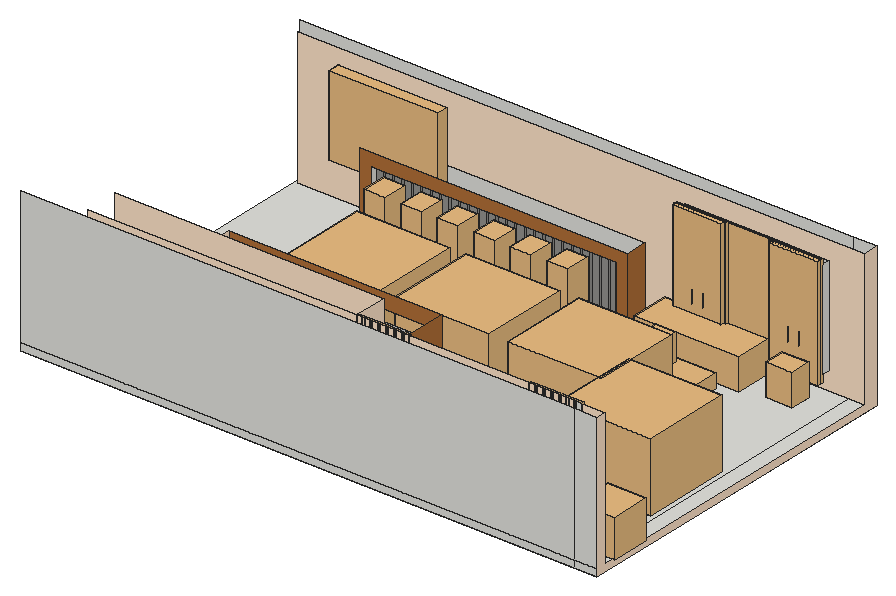
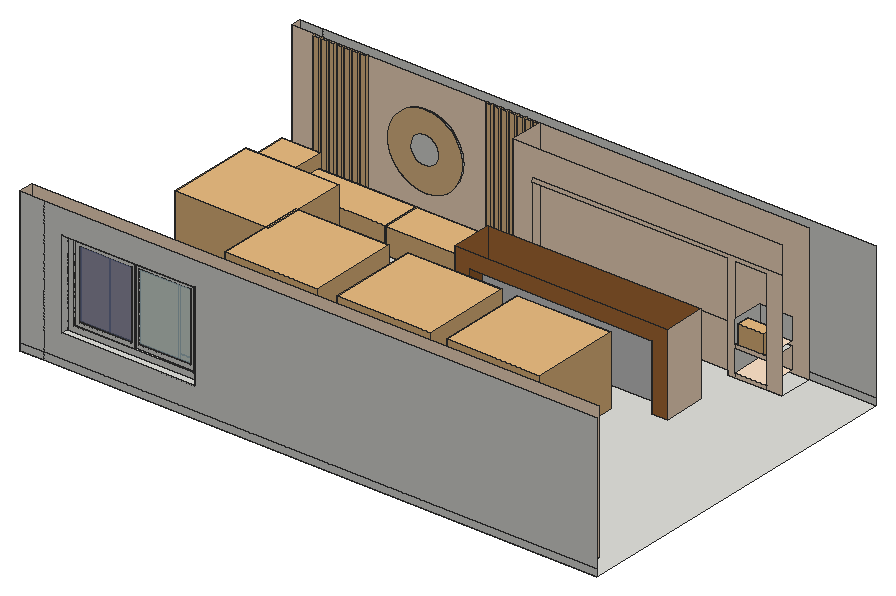
# SketchUp Ruby script. Lengths in inches.
U = 1.inch
M = Sketchup.active_model
def pt(a) = Geom::Point3d.new(a.map { |v| v * U })
def face(e, loops, mat)
  f = e.add_face(loops[0].map { |a| pt(a) })
  loops[1..].each { |l| e.add_face(l.map { |a| pt(a) }).erase! }
  f.material = f.back_material = mat if mat
  f
end
# faces: each face lists its corners as indices into pts; further lists are holes
def faces(e, pts, list, mat = nil) = list.each { |f| face(e, (f[0].is_a?(Array) ? f : [f]).map { |l| l.map { |i| pts[i] } }, mat) }
# xy, xz, yz: faces in a plane at the given z, y or x. An outline is a flat list of corners, or four numbers for a rectangle; further outlines are holes
def ring(l) = l.size == 4 ? [[l[0], l[1]], [l[2], l[1]], [l[2], l[3]], [l[0], l[3]]] : l.each_slice(2).to_a
def flat(e, list, mat, &to3) = list.each { |f| face(e, (f[0].is_a?(Array) ? f : [f]).map { |l| ring(l).map { |u, v| to3.(u, v) } }, mat) }
def xy(e, z, list, mat = nil) = flat(e, list, mat) { |x, y| [x, y, z] }
def xz(e, y, list, mat = nil) = flat(e, list, mat) { |x, z| [x, y, z] }
def yz(e, x, list, mat = nil) = flat(e, list, mat) { |y, z| [x, y, z] }
def lines(e, pts, list) = list.each { |a, b| e.add_line(pt(pts[a]), pt(pts[b])) }
# prism: a flat outline (further loops are holes) pulled along v
def prism(e, loops, v, mat = nil)
  f = face(e, loops, mat); d = Geom::Vector3d.new(v.map { |x| x * U })
  f.pushpull(f.normal.samedirection?(d) ? d.length : -d.length)
end
def box(e, o, s, mat = nil) = prism(e, [[o, [o[0] + s[0], o[1], o[2]], [o[0] + s[0], o[1] + s[1], o[2]], [o[0], o[1] + s[1], o[2]]]], [0, 0, s[2]], mat)
def at(x, y, z, deg = 0) = Geom::Transformation.translation(pt([x, y, z])) * Geom::Transformation.rotation(ORIGIN, Z_AXIS, deg.degrees)
def axes(o, x, y, z) = Geom::Transformation.new([*x, 0, *y, 0, *z, 0, *pt(o).to_a, 1])
def part(name) = M.definitions.add(name)
# library, detail: a bought-in or finely detailed component or shape, given as its bounding box
def library(name, o, s) = part(name).tap { |d| box(d.entities, o, s) }
def detail(e, o, s) = box(e.add_group.entities, o, s)
def put(e, d, t, mat = nil) = e.add_instance(d, t).tap { |i| i.material = mat if mat }
def group(e, t, mat = nil) = e.add_group.tap { |g| g.transformation = t; g.material = mat if mat }.entities
root = M.entities
M.materials.add("[Carrera Marble]").color = [207, 207, 207]
M.materials.add("[Color C02]").color = [255, 228, 201]
M.materials.add("[Granite Light Gray]").color = [149, 148, 144]
M.materials.add("[Translucent_Glass_Safety]").color = [204, 235, 244]
M.materials["[Translucent_Glass_Safety]"].alpha = 0.5
M.materials.add("[Translucent_Glass_Sky_Reflection]").color = [125, 138, 183]
M.materials["[Translucent_Glass_Sky_Reflection]"].alpha = 0.52
M.materials.add("[Wood Bamboo]").color = [177, 112, 56]
M.materials.add("[Wood Floor Dark]").color = [153, 94, 42]
M.materials.add("images").color = [235, 194, 141]
c1 = library("Group\#234",[0,0,0],[22.58,10.85,16.9375])
c2 = library("D\#1",[0,-5.78,0],[96.19,12.38,70.4375])
c3 = part("Group\#53")
xz(c3.entities,0,[[0,0,6.375,49.79]])
yz(c3.entities,6.375,[[0,0,2.75,49.79]])
c4 = library("bar+stool",[0,0,0],[13.78,17.63,39.8])
c5 = library("Group\#71",[0,0,0],[82.62,78.29,61.04])
c6 = part("Group\#54")
xz(c6.entities,2,[[0,0,5,120]])
yz(c6.entities,0,[[0,0,2,120]])
yz(c6.entities,5,[[0,0,2,120]])
c7 = library("Group\#57",[0,0,0],[112.99,39.26,34.22])
c8 = library("flower",[-43.13,-13.95,0.26],[17.98,19.13,23.85])
c9 = library("25984",[-0.01,-37.35,0],[37.87,32.46,16.84])
c10 = library("sofa+blue",[10.44,18.33,0.01],[94.56,54.06,43.33])
c11 = library("Group14",[-64.97,9.24,0.31],[138.52,9.93,292.57])
c12 = library("Group16",[86.37,-10.76,76.46],[21.79,14.87,35.97])
c13 = library("Group22",[48.82,-10.91,0.23],[97.72,18.57,293.12])
c14 = library("Group24",[44.03,2.01,0.26],[103.73,11,292.35])
c15 = library("Group27",[-106.21,-10.76,76.46],[21.8,14.87,35.97])
c16 = library("Group35",[-145.81,2.01,0.26],[103.73,11,292.35])
c17 = library("Group33",[-144.59,-10.91,0.23],[97.72,18.57,293.12])
c18 = part("rem")
g1 = group(c18.entities,at(-145.81,-10.91,0.23))
put(g1,c11,at(145.81,10.91,-0.23))
put(g1,c12,at(145.81,10.91,-0.23))
put(g1,c13,at(145.81,10.91,-0.23))
put(g1,c14,at(145.81,10.91,-0.23))
put(g1,c15,at(145.81,10.91,-0.23))
put(g1,c16,at(145.81,10.91,-0.23))
put(g1,c17,at(145.81,10.91,-0.23))
c19 = library("Untitled (7)",[0,0,0],[82.62,78.29,61.04])
c20 = library("Component\#7",[1.65,0,0],[13.63,13.63,20.73])
c21 = library("plants",[-0.26,-0.03,0],[11.57,13.37,22.79])
xy(root,-6,[[174.82,0,664.13,308.75],[664.13,0,684.57,308.75]])
xy(root,0,[[227.2,9,464.82,9,464.82,38.75,448.07,38.75,448.07,30,275.2,30,275.2,38.75,227.2,38.75],[659.13,9,664.13,11],[664.13,9,684.57,11]])
xy(root,3.75,[[275.2,30,448.07,38.75]])
xy(root,3.75,[[240.38,11.0625,269.2,38.75]],"[Color C02]")
xy(root,15.75,[[525.75,289.72,652.62,295.72]])
xy(root,20.44,[[530.43,289.72,647.93,295.72],[530.43,295.72,647.93,308.75]])
xy(root,23.0625,[[240.38,11.0625,269.2,38.75]])
xy(root,26.8125,[[240.38,11.0625,269.2,38.75]],"[Color C02]")
xz(root,0,[[174.82,-6,664.13,0],[664.13,-6,684.57,0],[174.82,0,664.13,120],[664.13,0,684.57,120]])
xz(root,9,[[659.13,0,664.13,120]])
xz(root,9,[[227.2,0,464.82,120],[[464.82,0,659.13,120],[566.46,30.45,570.25,30.89,573.96,31.76,577.55,33.05,580.96,34.76,584.16,36.85,587.09,39.29,589.71,42.0625,592,45.12,593.91,48.42,595.43,51.92,596.54,55.57,597.21,59.33,597.4375,63.14,597.23,66.95,596.57,70.71,595.49,74.36,593.98,77.87,592.08,81.18,589.8125,84.25,587.2,87.03,584.28,89.49,581.1,91.59,577.69,93.3125,574.11,94.625,570.4,95.51,566.61,95.97,562.8,95.98,559,95.54,555.29,94.67,551.7,93.375,548.29,91.67,545.09,89.58,542.17,87.13,539.54,84.37,537.25,81.31,535.34,78.01,533.82,74.51,532.72,70.86,532.04,67.1,531.8125,63.29,532.03,59.48,532.68,55.72,533.77,52.06,535.27,48.56,537.17,45.25,539.44,42.18,542.05,39.4,544.97,36.94,548.15,34.84,551.56,33.12,555.14,31.8,558.85,30.91,562.64,30.46]],[664.13,0,684.57,120]],"[Color C02]")
xz(root,11.0625,[[240.38,26.8125,269.2,46.125]])
xz(root,11.0625,[[240.38,3.75,269.2,23.0625]],"[Color C02]")
xz(root,11.5,[[[566.46,30.45,562.64,30.46,558.85,30.91,555.14,31.8,551.56,33.12,548.15,34.84,544.97,36.94,542.05,39.4,539.44,42.18,537.17,45.25,535.27,48.56,533.77,52.06,532.68,55.72,532.03,59.48,531.8125,63.29,532.04,67.1,532.72,70.86,533.82,74.51,535.34,78.01,537.25,81.31,539.54,84.37,542.17,87.13,545.09,89.58,548.29,91.67,551.7,93.375,555.29,94.67,559,95.54,562.8,95.98,566.61,95.97,570.4,95.51,574.11,94.625,577.69,93.3125,581.1,91.59,584.28,89.49,587.2,87.03,589.8125,84.25,592.08,81.18,593.98,77.87,595.49,74.36,596.57,70.71,597.23,66.95,597.4375,63.14,597.21,59.33,596.54,55.57,595.43,51.92,593.91,48.42,592,45.12,589.71,42.0625,587.09,39.29,584.16,36.85,580.96,34.76,577.55,33.05,573.96,31.76,570.25,30.89],[564.08,51.67,567.38,51.86,570.52,52.89,573.28,54.7,575.48,57.17,576.97,60.12,577.65,63.35,577.46,66.65,576.42,69.79,574.61,72.55,572.15,74.75,569.2,76.24,565.96,76.91,562.66,76.73,559.53,75.69,556.76,73.88,554.5625,71.42,553.08,68.47,552.4,65.23,552.59,61.93,553.625,58.8,555.44,56.03,557.9,53.83,560.85,52.35]]],"images")
xz(root,30,[[275.2,0,448.07,3.75]])
xz(root,38.75,[[227.2,0,227.2,96,448.07,96,448.07,92.25,275.2,92.25,275.2,0,269.2,0,269.2,92.25,240.38,92.25,240.38,0],[448.07,0,448.07,96,227.2,96,227.2,120,464.82,120,464.82,0],[240.38,0,269.2,3.75],[275.2,3.75,448.07,42.97],[240.38,23.0625,269.2,26.8125]],"[Color C02]")
xz(root,77.03,[[268.13,0,456.63,71.375]],"[Wood Bamboo]")
xz(root,100.22,[[281.8,0,442.97,57.71]],"[Carrera Marble]")
xz(root,113.97,[[268.13,0,268.13,71.375,456.63,71.375,456.63,0,442.97,0,442.97,57.71,281.8,57.71,281.8,0]],"[Wood Bamboo]")
xz(root,276.18,[[253.81,0,264.58,0,264.58,49.79,480.22,49.79,480.22,0,490.99,0,490.99,60.5625,253.81,60.5625]],"[Wood Bamboo]")
xz(root,283.81,[[270.96,0,480.22,49.79]])
xz(root,289.72,[[[525.75,15.75,652.62,103.32],[530.43,20.44,647.93,98.63]]])
xz(root,295.25,[[253.81,0,490.99,60.5625]])
xz(root,295.72,[[[525.75,15.75,652.62,103.32],[530.43,20.44,647.93,98.63]]])
xz(root,295.72,[[[183.82,0,684.57,120],[525.75,15.75,652.62,103.32]]],"[Color C02]")
xz(root,308.75,[[174.82,-6,664.13,0],[664.13,-6,684.57,0],[[174.82,0,664.13,120],[530.43,20.44,647.93,98.63]],[664.13,0,684.57,120]])
yz(root,264.58,[[276.18,0,281.06,49.79]])
yz(root,268.13,[[77.03,0,113.97,71.375]],"[Color C02]")
yz(root,269.2,[[11.0625,3.75,38.75,23.0625],[11.0625,26.8125,38.75,46.125]])
yz(root,275.2,[[30,0,38.75,3.75]])
yz(root,281.8,[[100.22,0,113.97,57.71]],"[Wood Bamboo]")
yz(root,442.97,[[100.22,0,113.97,57.71]],"[Wood Floor Dark]")
yz(root,448.07,[[30,0,38.75,3.75]])
yz(root,456.63,[[77.03,0,113.97,71.375]],"[Wood Bamboo]")
yz(root,464.82,[[9,0,38.75,120]],"[Color C02]")
yz(root,480.22,[[276.18,0,283.81,49.79]])
yz(root,490.99,[[276.18,0,295.25,60.5625]],"[Wood Bamboo]")
yz(root,525.75,[[289.72,15.75,295.72,103.32]])
yz(root,530.43,[[289.72,20.44,295.72,98.63],[295.72,20.44,308.75,98.63]])
yz(root,647.93,[[289.72,20.44,295.72,98.63],[295.72,20.44,308.75,98.63]])
yz(root,652.62,[[289.72,15.75,295.72,103.32]])
yz(root,684.57,[[0,-6,308.75,-6,308.75,120,295.72,120,295.72,0,9,0,9,120,0,120]],"[Color C02]")
p = [[562.64,9,30.46],[558.85,9,30.91],[558.85,11.5,30.91],[562.64,11.5,30.46],[566.46,9,30.45],[566.46,11.5,30.45],
  [570.25,9,30.89],[570.25,11.5,30.89],[555.14,9,31.8],[555.14,11.5,31.8],[573.96,9,31.76],[573.96,11.5,31.76],
  [551.56,9,33.12],[551.56,11.5,33.12],[577.55,9,33.05],[577.55,11.5,33.05],[548.15,9,34.84],[548.15,11.5,34.84],
  [580.96,9,34.76],[580.96,11.5,34.76],[544.97,9,36.94],[544.97,11.5,36.94],[584.16,9,36.85],[584.16,11.5,36.85],
  [587.09,9,39.29],[587.09,11.5,39.29],[542.05,9,39.4],[542.05,11.5,39.4]]
faces(root,p,[[0,1,2,3],[4,0,3,5],[6,4,5,7],[1,8,9,2],[10,6,7,11],[8,12,13,9],[14,10,11,15],[12,16,17,13],
  [18,14,15,19],[16,20,21,17],[22,18,19,23],[24,22,23,25],[20,26,27,21]],"images")
put(root,c1,at(243.55,27.9,26.8125))
put(root,c2,at(219.38,290.72,35.71))
put(root,c3,at(264.58,281.06,0),"[Granite Light Gray]")
put(root,c3,at(272.89,281.06,0),"[Granite Light Gray]")
put(root,c3,at(281.21,281.06,0),"[Granite Light Gray]")
put(root,c4,axes([294.6,275.52,0.78],[-1.356,0,0],[0,-1.243,0],[0,0,1.13]))
put(root,c3,at(289.52,281.06,0),"[Granite Light Gray]")
put(root,c3,at(297.83,281.06,0),"[Granite Light Gray]")
put(root,c3,at(306.14,281.06,0),"[Granite Light Gray]")
put(root,c4,axes([326.85,275.52,0.78],[-1.356,0,0],[0,-1.243,0],[0,0,1.13]))
put(root,c3,at(314.46,281.06,0),"[Granite Light Gray]")
put(root,c3,at(322.77,281.06,0),"[Granite Light Gray]")
put(root,c3,at(331.08,281.06,0),"[Granite Light Gray]")
put(root,c3,at(339.39,281.06,0),"[Granite Light Gray]")
put(root,c5,at(308,126.98,0))
put(root,c4,axes([359.1,275.52,0.78],[-1.356,0,0],[0,-1.243,0],[0,0,1.13]))
put(root,c3,at(347.71,281.06,0),"[Granite Light Gray]")
put(root,c3,at(356.02,281.06,0),"[Granite Light Gray]")
put(root,c3,at(364.33,281.06,0),"[Granite Light Gray]")
put(root,c3,at(372.64,281.06,0),"[Granite Light Gray]")
put(root,c4,axes([391.35,275.52,0.78],[-1.356,0,0],[0,-1.243,0],[0,0,1.13]))
put(root,c3,at(380.96,281.06,0),"[Granite Light Gray]")
put(root,c3,at(389.27,281.06,0),"[Granite Light Gray]")
put(root,c3,at(397.58,281.06,0),"[Granite Light Gray]")
put(root,c3,at(405.89,281.06,0),"[Granite Light Gray]")
put(root,c4,axes([423.6,275.52,0.78],[-1.356,0,0],[0,-1.243,0],[0,0,1.13]))
put(root,c3,at(414.21,281.06,0),"[Granite Light Gray]")
put(root,c3,at(422.52,281.06,0),"[Granite Light Gray]")
put(root,c3,at(430.83,281.06,0),"[Granite Light Gray]")
put(root,c3,at(439.14,281.06,0),"[Granite Light Gray]")
put(root,c5,at(404.625,126.98,0))
put(root,c4,axes([455.85,275.52,0.78],[-1.356,0,0],[0,-1.243,0],[0,0,1.13]))
put(root,c3,at(447.46,281.06,0),"[Granite Light Gray]")
put(root,c3,at(455.77,281.06,0),"[Granite Light Gray]")
put(root,c3,at(464.08,281.06,0),"[Granite Light Gray]")
put(root,c6,at(464.82,9,0),"images")
put(root,c6,at(471.76,9,0),"images")
put(root,c3,at(472.39,281.06,0),"[Granite Light Gray]")
put(root,c6,at(478.7,9,0),"images")
put(root,c3,at(480.71,281.06,0))
put(root,c6,at(485.63,9,0),"images")
put(root,c6,at(492.57,9,0),"images")
put(root,c6,at(499.51,9,0),"images")
put(root,c6,at(506.45,9,0),"images")
put(root,c7,axes([565.38,54.44,0],[-0.86,0,0],[0,-0.86,0],[0,0,0.6794]))
put(root,c5,at(504.0625,126.98,0))
put(root,c8,at(584.08,239.16,12.13))
put(root,c9,axes([524.71,254.5,0],[1.73,0,0],[0,1,0],[0,0,0.74]))
put(root,c10,axes([502.69,243.62,0],[0.9792,0,0],[0,0.64,0],[0,0,0.64]))
put(root,c18,axes([587.49,286.69,9.02],[0.44078,0,0],[0,0.21468,0],[0,0,0.33456]))
g2 = group(root,at(530.43,302.23,20.44))
xy(g2,0,[[0,-4.33,117.5,0]])
xy(g2,5.21,[[5.83,-4.33,58.75,-3.15],[58.75,-4.33,111.67,-2.36],[58.75,-2.36,111.67,-0.82],[5.83,-2,58.75,0],[58.75,-0.82,111.67,0]])
xy(g2,8.9375,[[10,-3.15,55.83,-2.76],[10,-2.4,55.83,-2],[61.67,-2.36,107.5,-1.97],[61.67,-1.22,107.5,-0.82]])
xy(g2,69.25,[[10,-3.15,55.83,-2.76],[10,-2.4,55.83,-2],[61.67,-2.36,107.5,-1.97],[61.67,-1.22,107.5,-0.82]])
xy(g2,72.98,[[5.83,-4.33,58.75,-3.15],[58.75,-4.33,111.67,-2.36],[58.75,-2.36,111.67,-0.82],[5.83,-2,58.75,0],[58.75,-0.82,111.67,0]])
xy(g2,78.1875,[[0,-4.33,117.5,0]])
xz(g2,-4.33,[[[0,0,117.5,78.1875],[5.83,5.21,111.67,72.98]]])
xz(g2,-3.15,[[[5.83,5.21,58.75,72.98],[10,8.9375,55.83,69.25]]])
xz(g2,-2.76,[[10,8.9375,55.83,69.25]],"[Translucent_Glass_Safety]")
xz(g2,-2.4,[[10,8.9375,55.83,69.25]],"[Translucent_Glass_Safety]")
xz(g2,-2.36,[[[58.75,5.21,111.67,72.98],[61.67,8.9375,107.5,69.25]]])
xz(g2,-2,[[[5.83,5.21,58.75,72.98],[10,8.9375,55.83,69.25]]])
xz(g2,-1.97,[[61.67,8.9375,107.5,69.25]],"[Translucent_Glass_Sky_Reflection]")
xz(g2,-1.22,[[61.67,8.9375,107.5,69.25]],"[Translucent_Glass_Sky_Reflection]")
xz(g2,-0.82,[[[58.75,5.21,111.67,72.98],[61.67,8.9375,107.5,69.25]]])
xz(g2,0,[[[0,0,117.5,78.1875],[5.83,5.21,111.67,72.98]]])
yz(g2,0,[[-4.33,0,0,78.1875]])
yz(g2,5.83,[[-4.33,5.21,-3.15,72.98],[-2,5.21,0,72.98]])
yz(g2,10,[[-3.15,8.9375,-2.76,69.25],[-2.4,8.9375,-2,69.25]])
yz(g2,55.83,[[-3.15,8.9375,-2.76,69.25],[-2.4,8.9375,-2,69.25]])
yz(g2,58.75,[[-3.15,5.21,-2.36,72.98],[-2.36,5.21,-2,72.98],[-2,5.21,-0.82,72.98]])
yz(g2,61.67,[[-2.36,8.9375,-1.97,69.25],[-1.22,8.9375,-0.82,69.25]])
yz(g2,107.5,[[-2.36,8.9375,-1.97,69.25],[-1.22,8.9375,-0.82,69.25]])
yz(g2,111.67,[[-4.33,5.21,-2.36,72.98],[-2.36,5.21,-0.82,72.98],[-0.82,5.21,0,72.98]])
yz(g2,117.5,[[-4.33,0,0,78.1875]])
put(root,c7,axes([661.69,54.44,0],[-0.86,0,0],[0,-0.86,0],[0,0,0.6794]))
put(root,c6,at(617.51,9,0),"images")
put(root,c19,at(584.3,81.96,0))
put(root,c6,at(624.45,9,0),"images")
put(root,c6,at(631.38,9,0),"images")
put(root,c20,axes([621.6,261.64,0],[1.7018,0,0],[0,1.34,0],[0,0,1.34]))
put(root,c6,at(638.32,9,0),"images")
put(root,c6,at(645.26,9,0),"images")
put(root,c6,at(652.2,9,0),"images")
put(root,c6,at(659.13,9,0),"images")
put(root,c21,axes([652.93,17.17,0],[2.95574,0,0],[0,2.62465,0],[0,0,1.48285]))
